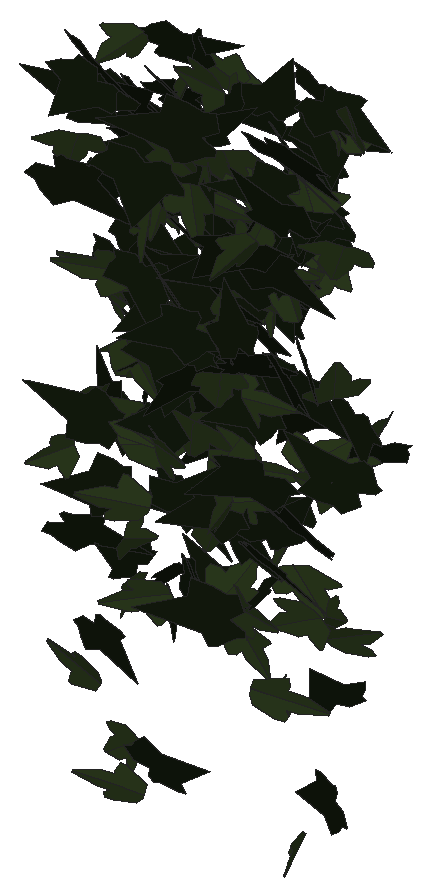
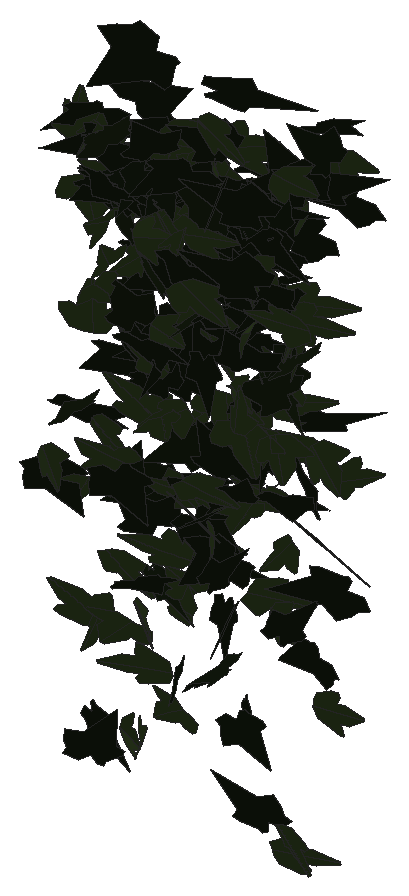
# SketchUp Ruby script. Lengths in millimetres.
U = 1.mm
M = Sketchup.active_model
def pt(a) = Geom::Point3d.new(a.map { |v| v * U })
def face(e, loops, mat)
  f = e.add_face(loops[0].map { |a| pt(a) })
  loops[1..].each { |l| e.add_face(l.map { |a| pt(a) }).erase! }
  f.material = f.back_material = mat if mat
  f
end
# faces: each face lists its corners as indices into pts; further lists are holes
def faces(e, pts, list, mat = nil) = list.each { |f| face(e, (f[0].is_a?(Array) ? f : [f]).map { |l| l.map { |i| pts[i] } }, mat) }
# xy, xz, yz: faces in a plane at the given z, y or x. An outline is a flat list of corners, or four numbers for a rectangle; further outlines are holes
def ring(l) = l.size == 4 ? [[l[0], l[1]], [l[2], l[1]], [l[2], l[3]], [l[0], l[3]]] : l.each_slice(2).to_a
def flat(e, list, mat, &to3) = list.each { |f| face(e, (f[0].is_a?(Array) ? f : [f]).map { |l| ring(l).map { |u, v| to3.(u, v) } }, mat) }
def xy(e, z, list, mat = nil) = flat(e, list, mat) { |x, y| [x, y, z] }
def xz(e, y, list, mat = nil) = flat(e, list, mat) { |x, z| [x, y, z] }
def yz(e, x, list, mat = nil) = flat(e, list, mat) { |y, z| [x, y, z] }
def lines(e, pts, list) = list.each { |a, b| e.add_line(pt(pts[a]), pt(pts[b])) }
# prism: a flat outline (further loops are holes) pulled along v
def prism(e, loops, v, mat = nil)
  f = face(e, loops, mat); d = Geom::Vector3d.new(v.map { |x| x * U })
  f.pushpull(f.normal.samedirection?(d) ? d.length : -d.length)
end
def box(e, o, s, mat = nil) = prism(e, [[o, [o[0] + s[0], o[1], o[2]], [o[0] + s[0], o[1] + s[1], o[2]], [o[0], o[1] + s[1], o[2]]]], [0, 0, s[2]], mat)
def at(x, y, z, deg = 0) = Geom::Transformation.translation(pt([x, y, z])) * Geom::Transformation.rotation(ORIGIN, Z_AXIS, deg.degrees)
def axes(o, x, y, z) = Geom::Transformation.new([*x, 0, *y, 0, *z, 0, *pt(o).to_a, 1])
def part(name) = M.definitions.add(name)
# library, detail: a bought-in or finely detailed component or shape, given as its bounding box
def library(name, o, s) = part(name).tap { |d| box(d.entities, o, s) }
def detail(e, o, s) = box(e.add_group.entities, o, s)
def put(e, d, t, mat = nil) = e.add_instance(d, t).tap { |i| i.material = mat if mat }
def group(e, t, mat = nil) = e.add_group.tap { |g| g.transformation = t; g.material = mat if mat }.entities
root = M.entities
M.materials.add("efeu1").color = [18, 25, 13]
M.materials.add("efeu2").color = [43, 57, 29]
c1 = part("ivyleaf_10")
p = [[0,12.8,-0.8],[-1.5,51.3,-10.9],[-4.9,51,-11.6],[-13.6,26.5,-7.3],[-13.2,15.9,-4.6],[-21.1,19.3,-7.2],
  [-29.5,16.3,-8.3],[-29.2,8.3,-6.2],[-19.7,-9.8,0.5],[-7.6,-13,4],[1,-12.2,5.8],[-0.4,51.1,-11.1],
  [-1.5,51.1,-10.9],[1,-12.4,5.9],[16.9,-12.4,3.5],[35.1,9.1,-5.1],[35,12.9,-6.1],[20.5,16.4,-4.9],
  [15.8,15,-3.8],[15.3,27.6,-7.1],[12.8,31.3,-7.8]]
faces(c1.entities,p,[[0,1,2,3,4,5,6,7,8,9,10],[11,12,0,13,14,15,16,17,18,19,20]],"efeu2")
c2 = part("ivyleaf_9")
p = [[39.1,54.8,31.7],[34.5,51.8,30.2],[-5.3,25.2,17.3],[-17.9,28.3,20.9],[-21.6,21.7,17],[-20.2,4.3,5.3],
  [-22.9,-0.3,2.5],[-17.1,-4,-0.6],[-2,-2.1,-1.2],[-0.7,-15.4,-10.1],[16.6,-22.3,-16.7],[21.1,-15.1,-12.5],
  [32.7,-10.7,-11],[46.1,-1.8,-6.6],[30.8,11.2,3.8]]
faces(c2.entities,p,[[0,1,2,3,4,5,6,7,8,9,10,11,12,13,14]],"efeu1")
put(root,c1,axes([3959.3,865.1,1629.4],[-0.5188,-0.54875,0.84407],[-0.22094,-0.8515,-0.59107],[1.90331,-0.24842,0.16146]))
put(root,c1,axes([3980.2,743.2,691],[-0.45175,0.21284,-0.91602],[-1.44478,0.51427,0.3162],[1.05644,0.79433,0.04073]))
put(root,c1,axes([3965.8,850.5,533.4],[1.04762,-0.60703,-0.60546],[-0.73059,0.46885,-0.81907],[1.45903,0.67064,0.02459]))
put(root,c1,axes([3920,890.6,1409.7],[-0.39414,-0.01153,-0.95363],[1.73672,-0.28603,-0.19471],[-0.52755,-0.933,0.07148]))
put(root,c2,axes([3991.9,777.8,1569.6],[-0.28849,0.0607,1.14922],[-2.18862,-0.05262,-0.1489],[0.08433,-1.15798,0.06701]))
put(root,c2,axes([3975.1,796.3,1081.1],[0.12478,0.00613,1.16954],[-0.12199,1.16963,-0.00254],[-2.22255,-0.06386,0.0658]))
put(root,c2,axes([3971.7,955.8,765.4],[-0.31084,0.75727,-0.51997],[0.19505,-0.5098,-0.77466],[-1.73736,-0.19272,0.00606]))
put(root,c1,axes([3972.5,705.2,1058.3],[0.21292,0.15716,-1.04889],[-0.94197,-0.92508,-0.1914],[-1.78526,0.50685,-0.0241]))
put(root,c1,axes([3990.2,821.5,481.6],[0.24968,0.09856,0.91362],[-1.44052,-0.51174,0.16389],[0.99172,-0.76814,0.00805]))
put(root,c1,axes([3973.4,764.7,1120.4],[-0.19767,-1.14603,0.30004],[-0.0368,-0.29951,-1.1507],[2.25434,-0.10538,0.00753]))
put(root,c1,axes([3970.4,827.9,1355.5],[0.48526,-0.30388,-1.02495],[0.00398,1.05383,-0.31193],[2.03461,0.07042,0.24507]))
put(root,c2,axes([3937.3,754.8,906.7],[0.32283,0.21121,-0.96973],[0.96693,0.82663,0.26891],[1.6226,-0.53463,0.03269]))
put(root,c2,axes([3944.2,782.7,1631.3],[0.53927,-0.56852,0.83965],[0.67816,-0.76039,-0.6351],[1.80678,0.45509,-0.01223]))
put(root,c2,axes([4014.9,757.6,987.8],[-1.56685,0.75225,0.36065],[-0.55985,0.21237,-1.11449],[-1.48572,-0.87335,0.03962]))
put(root,c1,axes([3986,845.9,1170.5],[-0.89079,-0.97271,-0.03245],[0.05811,0.02131,-1.07931],[1.85138,-0.46869,0.01827]))
put(root,c1,axes([3987.7,892.9,1483.1],[-0.11806,-0.85719,0.53445],[0.0114,-0.53576,-0.8586],[1.9225,-0.04946,0.03791]))
put(root,c2,axes([3966,828.1,1304.4],[0.14063,-1.03369,0.34224],[0.08121,-0.34001,-1.03619],[2.07076,0.08354,0.01739]))
put(root,c2,axes([3973.7,899,1446.5],[-1.18222,0.17725,0.73217],[1.18572,-0.41261,0.62845],[0.80599,0.867,0.1494]))
put(root,c2,axes([3950.4,953.6,1498.3],[0.57315,-0.22264,0.87712],[1.71725,0.00334,-0.30895],[0.13142,0.92737,0.21169]))
put(root,c1,axes([4024.5,759.8,1327.3],[-0.16228,0.03151,-1.04796],[-1.99092,-0.07288,0.08292],[-0.13345,1.0489,0.03725]))
put(root,c2,axes([3985.2,830,1076.9],[-1.15832,-0.62712,-0.2686],[0.35475,0.19339,-0.8739],[1.249,-0.63652,-0.00089]))
put(root,c1,axes([4002.9,904.7,1473.6],[0.31414,-0.4115,-0.84591],[-0.55598,0.79395,-0.44322],[1.7018,0.33534,0.01135]))
put(root,c2,axes([4022.5,859.4,1518.9],[0.01221,0.09272,-1.01055],[-1.83432,-0.31575,-0.03509],[-0.6045,0.95998,0.08606]))
put(root,c2,axes([4002.3,818.7,839.9],[0.25264,0.09874,0.93701],[-1.38172,-0.59242,0.16528],[1.14297,-0.738,-0.00731]))
put(root,c2,axes([4000.5,982.4,1000.1],[0.03816,-0.01733,0.94339],[-1.19837,-0.703,0.00047],[1.33741,-0.62942,-0.0265]))
put(root,c2,axes([4014.4,884.1,743.2],[0.20682,0.00701,-0.96456],[-1.64727,0.42917,-0.09439],[0.81034,0.87063,0.0543]))
put(root,c1,axes([3986.6,916.8,1097.2],[0.736,0.88073,0.19755],[0.1551,0.17997,-0.96189],[-1.71084,0.3952,-0.00222]))
put(root,c2,axes([4007.7,723.2,1639.6],[-1.20806,-0.67927,0.40065],[-0.471,-0.31675,-0.92912],[1.42509,-0.68051,0.03256]))
put(root,c2,axes([3972.5,844.6,1498.5],[1.54358,0.26888,0.39363],[0.69227,0.15304,-0.85399],[-0.5864,0.88843,0.02797]))
put(root,c1,axes([4007.5,682.2,1566.9],[-1.41854,-0.74022,0.08376],[-0.11277,-0.05921,-1.05046],[1.41328,-0.7477,0.00026]))
put(root,c1,axes([4035.5,740.3,1344],[-0.03682,-0.00566,-1.13432],[-1.94851,-0.48838,0.0199],[-0.92952,1.02399,0.00322]))
put(root,c2,axes([3981.5,970.6,857.2],[0.86654,-0.8092,-0.15571],[-0.14488,0.13584,-0.92849],[1.56161,0.46162,0.00026]))
put(root,c1,axes([4010.8,762.3,1289.9],[-0.55669,0.59897,0.81223],[-0.69346,0.72593,-0.66655],[-1.79114,-0.46721,0.00562]))
put(root,c2,axes([3966.7,923.5,1595.4],[0.35313,-0.02317,0.97755],[1.85352,-0.08478,-0.18686],[0.16675,0.99139,0.00686]))
put(root,c2,axes([3974.5,801.1,1575.2],[2.06075,-0.09705,-0.23007],[0.45128,0.07867,1.08275],[-0.14898,-1.10415,0.09737]))
put(root,c1,axes([4017.1,880.4,1358.7],[0.00474,0.6236,-0.76732],[-0.28991,0.7584,0.61586],[1.85935,0.11666,0.09798]))
put(root,c2,axes([3983.6,856.4,1541.6],[0.11582,-0.4186,0.95953],[0.59879,-0.9094,-0.41669],[1.90028,0.31207,0.07282]))
put(root,c2,axes([4040.2,703.4,1127.9],[-1.0054,-0.84373,-0.40503],[-0.35276,-0.36157,0.99495],[-1.74595,0.55892,0.03221]))
put(root,c1,axes([4035.1,981.4,1148.1],[0.96134,0.24095,-0.77105],[-1.36113,-0.28945,-0.55897],[-0.71488,0.87514,0.02741]))
put(root,c2,axes([4027.6,817.5,1143.6],[0.01757,0.05,-1.03786],[-1.46352,0.69835,0.02681],[1.32996,0.76782,0.04321]))
put(root,c1,axes([4046.4,971,1551.7],[0.7857,0.08387,0.85888],[-1.59559,-0.1867,0.4212],[0.3893,-0.93448,-0.00706]))
put(root,c2,axes([3993.1,745,771],[-0.34449,-0.05084,-0.95511],[1.80333,0.12305,-0.18612],[0.24829,-0.96429,0.02661]))
put(root,c2,axes([3982.2,676.6,1511.3],[0.1515,-0.21733,-1.11977],[1.78305,0.65277,-0.06009],[1.23837,-0.91329,0.22351]))
put(root,c2,axes([3992.3,752.7,1479.1],[0.52878,0.29984,-0.99452],[0.71031,0.93192,0.38524],[1.84491,-0.44474,0.13673]))
put(root,c2,axes([4009.4,916,1091.5],[-0.27308,-0.21788,0.95466],[1.55252,0.50714,0.23835],[-1.03092,0.82145,0.10606]))
put(root,c2,axes([4013.2,799.1,1391.5],[0.42792,-0.41087,-1.00066],[-0.5291,0.96576,-0.45901],[1.98959,0.3452,0.09315]))
put(root,c2,axes([3992.6,881.6,1568.5],[1.50869,-0.67716,0.24411],[0.35844,-0.15536,-1.04255],[1.32222,0.81477,0.00409]))
put(root,c2,axes([4009.9,925,1009.6],[1.40511,0.54308,0.36462],[0.55207,0.22099,-0.9165],[-1.11583,0.79321,0.0057]))
put(root,c1,axes([4047.3,850.1,1171.6],[-2.10997,0.00574,0.38048],[-0.72416,-0.00251,-1.10865],[-0.00879,-1.17211,0.00423]))
put(root,c2,axes([3994.4,819.9,1241.7],[1.21504,-0.80467,0.3748],[0.50445,-0.2678,-1.02644],[1.61235,0.69017,0.03869]))
put(root,c2,axes([4020.4,981.5,1097.9],[-0.30074,-0.9049,0.23974],[-0.09171,-0.23495,-0.91856],[1.77925,-0.16506,-0.00683]))
put(root,c2,axes([4033.6,913.4,1613],[0.58197,-0.11355,-0.91049],[-1.26157,0.63625,-0.30197],[1.20744,0.7195,0.12334]))
put(root,c2,axes([4003.5,778,1264.8],[1.67676,-0.58861,-0.09034],[-0.12402,0.06506,-1.05941],[1.12656,0.88325,0.01784]))
put(root,c1,axes([4030.3,889,1567.8],[0.72251,-0.89473,0.17404],[0.15816,-0.15377,-0.9718],[1.72754,0.38828,0.01618]))
put(root,c2,axes([4059,801.5,1514.5],[-0.98542,-0.25859,0.76669],[-1.34808,-0.29511,-0.57789],[0.74435,-0.87682,-0.03161]))
put(root,c1,axes([4047.5,923.3,1025.3],[0.10702,-0.09961,0.98424],[-1.07951,0.80445,0.11382],[-1.54257,-0.56987,-0.01137]))
put(root,c1,axes([4003.9,744.4,1111.6],[0.93535,0.48869,0.89138],[1.18993,0.63537,-0.69305],[-1.52549,0.79524,0.00595]))
put(root,c1,axes([4035.6,785.5,839.4],[0.27271,-0.90028,0.5439],[0.25623,-0.52871,-0.91061],[1.98536,0.1919,0.04281]))
put(root,c2,axes([4058.5,758.6,1214.1],[-0.4518,0.92759,0.36764],[-0.17051,0.35656,-0.95748],[-1.89132,-0.25373,-0.0015]))
put(root,c1,axes([4024.3,747.9,1512.6],[-0.90522,0.829,-0.60657],[0.59387,-0.52025,-0.9557],[-1.86262,-0.56876,-0.00992]))
put(root,c1,axes([4035.4,875.9,1203],[-1.30905,0.62472,0.39731],[0.55759,-0.26837,0.92917],[1.29403,0.74761,0.00155]))
put(root,c2,axes([4034.2,855.2,1291.9],[-1.1481,-0.14236,0.71503],[1.3556,0.08292,0.61743],[-0.29603,0.93182,0.05429]))
put(root,c1,axes([4044,824.8,1156.3],[-1.55833,-0.68303,-0.25266],[0.37039,0.16114,-1.06628],[1.33562,-0.8416,0.0009]))
put(root,c2,axes([4072.6,921.7,777.9],[-0.79872,-0.82739,0.35569],[0.29237,0.3209,0.92771],[-1.68891,0.44684,-0.00762]))
put(root,c1,axes([4050.5,742.7,931.9],[-0.26613,-0.38674,-0.93422],[0.59974,0.87947,-0.41125],[1.82849,-0.34475,-0.00108]))
put(root,c2,axes([4025.7,825.2,526.5],[-0.01457,0.02402,0.95368],[1.32773,-0.65036,0.02198],[1.23839,0.69756,-0.01235]))
put(root,c1,axes([4052.1,808.4,1424.9],[1.18227,-0.77185,0.22562],[0.28592,-0.16868,-0.99072],[1.50351,0.63901,0.01099]))
put(root,c1,axes([4020.8,797.8,1043.3],[1.01431,-0.22774,-0.89789],[1.75743,0.0486,0.53577],[-0.13957,-1.04301,0.22102]))
put(root,c2,axes([4076,904.1,1301],[0.8911,-0.05599,-0.8817],[-1.63125,0.2132,-0.46869],[0.40776,0.97528,0.05184]))
put(root,c1,axes([4091.1,755,848.1],[0.54036,0.20306,-1.03576],[-1.59962,-0.60529,-0.34906],[-1.21508,0.88715,-0.00108]))
put(root,c1,axes([4065.8,969.7,1550.4],[0.23464,0.93867,-0.15253],[-0.06358,-0.14943,-0.94664],[-1.80879,0.12702,0.01349]))
put(root,c2,axes([4077.8,889.4,1554],[0.50407,0.77888,0.57502],[0.35612,0.54372,-0.82268],[-1.80783,0.32428,-0.00173]))
put(root,c2,axes([4053.5,807.6,1438.7],[-0.92735,0.16597,1.02057],[1.73071,-0.46816,0.5103],[0.93655,1.02947,0.06753]))
put(root,c2,axes([4092.2,900.2,1036.4],[-0.10703,0.43277,-0.84754],[0.06019,-0.84769,-0.43495],[-1.81015,-0.05378,0.03565]))
put(root,c1,axes([4045.7,750.8,1218],[1.30161,-0.27451,0.95007],[1.70821,-0.3127,-0.73644],[0.79024,1.12809,0.02706]))
put(root,c1,axes([4078.7,820.4,1088],[-0.58132,-0.87118,-0.03194],[-0.0202,-0.03012,0.92317],[-1.65901,0.30563,-0.00005]))
put(root,c2,axes([4087.5,911.1,1041.8],[-1.30778,0.71498,-0.02906],[-0.0586,0.01071,0.99154],[1.36062,0.68768,0.01477]))
put(root,c1,axes([4084.9,815.6,1212.4],[0.40159,-0.79797,0.49323],[0.29082,-0.46957,-0.82506],[1.76155,0.25944,0.02377]))
put(root,c2,axes([4087.3,823.6,849],[0.71431,-0.38393,-0.85916],[-1.14458,0.61358,-0.53691],[1.37753,0.7089,-0.0006]))
put(root,c1,axes([4113.7,893,1402.1],[-1.15489,-0.47004,0.63147],[-0.96006,-0.37991,-0.76754],[1.15017,-0.78908,-0.00661]))
put(root,c2,axes([4070.4,849.1,1097.7],[-0.89777,-0.03829,0.85441],[1.38276,-0.53275,0.37725],[0.85881,0.81775,0.28577]))
put(root,c2,axes([4103.5,821.8,852.7],[0.84581,-0.11014,-0.90603],[-1.6166,0.31882,-0.4554],[0.63559,0.95747,0.04741]))
put(root,c2,axes([4082.5,742,1362.8],[-0.50687,-1.07412,-0.0713],[0.04352,0.06779,-1.10662],[2.04829,-0.26724,0.00587]))
put(root,c2,axes([4098.8,765.6,1300],[0.21039,-0.41617,-1.00154],[0.46241,-0.97164,0.43056],[-2.01169,-0.26687,-0.00578]))
put(root,c2,axes([4073.2,773.6,1339.5],[-0.47434,0.02793,0.93591],[1.72672,-0.23219,0.24853],[0.44048,0.94028,0.03357]))
put(root,c1,axes([4085.3,736.5,1448.4],[1.02341,-0.67256,0.75229],[0.85409,-0.60411,-0.86086],[1.72014,0.7001,-0.02014]))
put(root,c2,axes([4096.9,718.3,1541.2],[-1.18243,-0.96049,-0.15125],[0.15929,0.126,-1.14391],[1.84366,-0.62689,0.00183]))
put(root,c1,axes([4097.5,977,1231.1],[0.66283,0.84637,-0.28373],[-0.20548,-0.26238,-0.91523],[-1.68644,0.36462,0]))
put(root,c1,axes([4133.7,819.6,1632.9],[0.50574,-0.19376,-1.04021],[-1.36764,0.75419,-0.32406],[1.47813,0.7641,0.05607]))
put(root,c2,axes([4108.7,788.4,999.5],[0.41984,-0.71775,-0.75354],[0.48759,-0.70912,0.75044],[-1.91964,-0.3371,0.02581]))
put(root,c2,axes([4129.4,876,1077.8],[-1.56644,-0.47534,0.30066],[-0.49927,-0.14695,-0.95045],[0.94689,-0.86384,-0.00376]))
put(root,c1,axes([4147.8,732.4,1559.2],[-1.19547,0.36275,-0.8921],[-1.46589,0.45013,0.72535],[1.10023,0.99387,-0.00291]))
put(root,c2,axes([4132.1,753.7,1135.3],[-0.57594,-0.34038,1.09723],[-1.40365,-0.81241,-0.45543],[1.67637,-0.79718,-0.00437]))
put(root,c2,axes([4101.6,934.9,777.7],[0.25375,-0.15782,-0.98314],[1.48344,-0.60072,0.20214],[-1.17928,-0.78961,0.04273]))
put(root,c1,axes([4135,829.2,948.9],[-1.2988,-0.84989,0.07287],[-0.08314,-0.05837,-1.08996],[1.62131,-0.68382,0.00248]))
put(root,c2,axes([4131.4,914.2,1333.9],[0.48913,-0.90153,-0.3941],[0.22067,-0.37674,0.93742],[-1.85953,-0.28185,0.00758]))
put(root,c1,axes([4132.7,937.3,1351.2],[-0.0358,-0.66501,0.68277],[0.01748,-0.683,-0.66498],[1.81387,-0.00654,0.01989]))
put(root,c2,axes([4124.3,710.3,1392.4],[1.40679,-0.3417,-0.62969],[-1.073,0.28083,-0.8142],[0.84133,0.92953,0.01451]))
put(root,c1,axes([4134.6,804.9,1270.4],[1.5576,-0.56988,-0.2026],[-0.29497,0.1319,-0.99709],[1.11266,0.83273,0.01929]))
put(root,c1,axes([4159.4,618.3,1076.9],[0.14102,0.27954,1.0388],[-0.94969,-0.91353,0.28142],[1.81379,-0.50005,0.06658]))
put(root,c1,axes([4109.6,919.9,719.5],[1.3014,-0.17805,0.68953],[1.2916,-0.1268,-0.70575],[0.41078,0.96278,0.03457]))
put(root,c1,axes([4142.6,856.8,1058.7],[1.8977,-0.36879,-0.24772],[-0.42754,0.10659,-1.06291],[0.72948,1.02188,0.02147]))
put(root,c2,axes([4110.3,800.8,1399.4],[1.60916,-0.26924,-0.63782],[1.12677,-0.24068,0.88642],[-0.683,-1.03139,-0.04035]))
put(root,c2,axes([4145.3,959.8,1336.7],[-1.58385,-0.32565,-0.35437],[0.63283,0.12271,-0.89363],[0.6622,-0.89615,0.00641]))
put(root,c1,axes([4111.6,925.4,980.3],[-0.37019,-0.09506,0.98352],[1.56689,0.5387,0.21489],[-1.03988,0.84555,-0.02633]))
put(root,c2,axes([4142.5,903.6,1292.6],[0.40633,-0.33568,-0.92615],[-0.93997,0.78348,-0.39782],[1.62221,0.53806,0.00147]))
put(root,c2,axes([4130.2,762.3,1520.7],[-0.4223,-0.87568,-0.56529],[0.3186,0.54052,-0.903],[1.95793,-0.27682,0.02501]))
put(root,c2,axes([4145.9,744.4,1251.9],[-1.57213,-0.82852,-0.24431],[0.33429,0.16986,-1.16995],[1.60961,-0.8445,0.00436]))
put(root,c1,axes([4119,722.1,1104.4],[-0.81597,0.09254,1.03856],[1.7009,-0.54581,0.41757],[1.02217,0.98209,0.13421]))
put(root,c1,axes([4159.8,752,1139.4],[-2.05521,-0.00447,0.20463],[-0.38938,-0.00803,-1.07986],[0.0112,-1.09906,0.00705]))
put(root,c2,axes([4162.4,803,1243.9],[0.33297,-0.63504,0.84748],[-0.25241,0.83907,0.65611],[-1.99964,-0.21166,0.0583]))
put(root,c2,axes([4125.5,877.3,1589.2],[-0.11988,-0.31077,-1.01968],[0.52624,0.98174,-0.31629],[1.95935,-0.28269,0.02256]))
put(root,c2,axes([4132.3,843.9,1332.8],[0.14937,-1.1817,-0.18202],[-0.02935,0.1814,-1.1843],[2.27535,0.07991,-0.00333]))
put(root,c2,axes([4157.7,959.1,935.4],[-1.05387,-0.77052,0.15859],[-0.17214,-0.13029,-0.94885],[1.48726,-0.56107,0.00255]))
put(root,c2,axes([4197.5,711.7,1625.2],[-1.33243,-0.05021,0.93375],[-1.76909,-0.08969,-0.70176],[0.19385,-1.16361,0.0138]))
put(root,c1,axes([4164.6,942.2,874.8],[0.69109,-0.90909,-0.12377],[-0.09415,0.11352,-0.97893],[1.74361,0.36646,-0.0038]))
put(root,c1,axes([4145.2,784.1,1497.5],[-1.37136,-0.22656,-0.62415],[1.12253,0.20465,-0.7552],[0.58043,-0.93106,-0.01412]))
put(root,c2,axes([4144.4,778.1,1579.3],[-0.05581,-0.01886,0.99555],[1.66718,0.47306,0.03476],[-0.90102,0.87647,0.00266]))
put(root,c2,axes([4154.2,842.2,1406],[-1.37944,-0.13793,-0.87148],[1.61477,0.20057,-0.73739],[0.46086,-1.11561,-0.02483]))
put(root,c2,axes([4161.1,728.1,1023.3],[-1.11741,-0.05013,0.79979],[1.51699,0.06588,0.58926],[-0.15753,0.98997,0.00129]))
put(root,c1,axes([4134.1,781,1483.3],[-0.0525,-0.06474,-1.11764],[2.0184,-0.35961,-0.00535],[-0.68247,-1.05857,0.07016]))
put(root,c1,axes([4160.9,857.5,1168.8],[-0.41114,-0.26819,-0.96426],[1.05518,0.78922,-0.34372],[1.58588,-0.59464,-0.02129]))
put(root,c2,axes([4149.4,846.1,1208.8],[-0.00512,-0.16357,0.98202],[0.88986,-0.86719,-0.14316],[1.67277,0.46082,0.07916]))
put(root,c1,axes([4154.4,780.4,1547.6],[0.18232,-0.09945,1.12868],[1.3919,-0.85972,-0.13782],[1.64706,0.73755,-0.00847]))
put(root,c1,axes([4165.4,818.2,857.9],[0.97125,0.60104,-0.65119],[0.8034,0.49583,0.78846],[1.4829,-0.66229,-0.00066]))
put(root,c2,axes([4222.7,741.9,865.4],[-1.62417,0.08103,0.70567],[-1.33677,0.06808,-0.85723],[-0.20141,-1.10527,-0.00107]))
put(root,c1,axes([4173.5,931.5,654.2],[-0.01833,0.24464,-0.92655],[0.10711,-0.92485,-0.24478],[-1.8207,-0.05687,-0.00507]))
put(root,c1,axes([4207.5,881.9,1454.2],[-0.64367,0.54046,-0.77229],[-1.0865,0.53546,0.62473],[1.42755,0.65122,0.12726]))
put(root,c2,axes([4195.5,705.3,1255],[-0.32404,0.68314,-0.9242],[0.33745,-0.90749,-0.70345],[-2.1611,-0.24413,0.02873]))
put(root,c2,axes([4157.2,889.4,1230.9],[0.27826,-0.34802,0.88683],[0.62463,-0.82389,-0.37743],[1.70213,0.35924,-0.00647]))
put(root,c2,axes([4170,835.6,946.5],[0.99524,-0.72251,-0.61524],[-0.60159,0.52973,-0.89076],[1.70293,0.60939,0.04488]))
put(root,c2,axes([4197.4,886.1,1410.5],[-1.32954,0.48635,-0.46952],[0.71273,-0.2837,-0.85104],[-1.07112,-0.79245,0.01651]))
put(root,c1,axes([4164.8,731,1511.6],[1.6932,-0.48685,0.6537],[1.08888,-0.31622,-1.01416],[1.10487,1.05775,-0.00231]))
put(root,c1,axes([4158,912.5,1275.5],[0.60157,-0.22187,-0.94561],[1.43474,-0.57099,0.38596],[-1.16561,-0.81734,-0.01294]))
put(root,c2,axes([4206.1,943.5,1088.8],[0.22107,0.74175,-0.59653],[-0.16495,-0.59022,-0.75077],[-1.80406,0.14486,-0.00445]))
put(root,c2,axes([4195.2,873.3,1598],[-0.82609,-0.33463,0.84206],[1.36391,0.44459,0.54608],[-1.05532,0.83654,0.04661]))
put(root,c2,axes([4204.3,744.9,1333.4],[-1.86316,-0.10643,0.69661],[1.31595,0.08506,0.9847],[-0.25886,1.1985,-0.00803]))
put(root,c2,axes([4221,833.6,869.8],[-0.98447,0.78347,-0.3447],[0.37744,-0.28209,-0.93878],[-1.58471,-0.5539,-0.00946]))
put(root,c1,axes([4207.8,759.1,1575.5],[-1.69086,-0.62522,-0.23962],[0.37213,0.13851,-1.08637],[1.21876,-0.90969,-0.00073]))
put(root,c1,axes([4173.6,827.3,825.8],[-0.45687,0.07296,1.05185],[1.91807,-0.30115,0.2509],[0.58973,1.03601,-0.00115]))
put(root,c2,axes([4174.4,763.7,1349.1],[0.55885,-0.36188,0.86209],[1.01084,-0.67909,-0.46597],[1.46443,0.60685,-0.00735]))
put(root,c1,axes([4178.7,808,1004.3],[0.53255,0.08284,-0.88496],[1.57603,0.31279,0.29112],[0.6146,-0.87386,0.02031]))
put(root,c2,axes([4191.5,778.9,1069.6],[1.67644,-0.42555,-0.01649],[-0.02114,0.01493,-0.97822],[0.81024,0.88088,0.00861]))
put(root,c2,axes([4199.1,894.7,1268.6],[-0.26301,0.21278,0.98147],[0.49471,-0.94938,0.24243],[1.8462,0.28471,0.07486]))
put(root,c1,axes([4225.1,724.2,1248.9],[-1.3056,-0.72851,-0.02067],[0.04,0.0086,-1.00062],[1.38648,-0.68626,0.00941]))
put(root,c2,axes([4190.9,803.4,1370.5],[1.88514,0.13202,0.2585],[0.48758,0.03452,-0.99927],[-0.2597,1.02311,0.00036]))
put(root,c2,axes([4235.5,720.8,1049.8],[-0.05563,-0.38443,-0.92473],[-0.10658,-0.92304,0.3855],[-1.90298,0.06294,0.00544]))
put(root,c1,axes([4195.9,933.3,837.7],[1.59402,0.30136,0.48768],[0.87272,0.16602,-0.89011],[-0.65482,0.95486,0.00085]))
put(root,c2,axes([4214.7,872.7,1554.9],[1.38483,-0.3147,-0.63293],[-1.05863,0.30558,-0.7914],[0.8301,0.9147,0.04663]))
put(root,c2,axes([4227.7,976,632.9],[0.8205,0.27712,0.8202],[-1.40467,-0.36131,0.51001],[0.86128,-0.85326,0.05042]))
put(root,c1,axes([4209,816,1406.6],[1.85511,-0.54995,-0.13311],[0.23046,-0.05626,1.11913],[-1.05195,-0.98217,0.01043]))
put(root,c2,axes([4191.4,790.1,1233.1],[1.47486,0.33465,0.69773],[1.20983,0.2878,-0.84406],[-0.83985,1.00226,0.0094]))
put(root,c2,axes([4237.6,800.8,1174.3],[0.07899,-0.51476,-0.88394],[0.07641,-0.88316,0.5162],[-1.94529,-0.05559,-0.01562]))
put(root,c2,axes([4200.9,910,1334.2],[-0.10661,-0.42556,0.89771],[0.80492,-0.8238,-0.36413],[1.71088,0.36106,0.22725]))
put(root,c2,axes([4246.5,638.8,1372.3],[-0.25671,-0.4355,-0.98711],[-0.05877,-0.99283,0.44225],[-2.05255,0.08289,0.11079]))
put(root,c2,axes([4242.7,853.1,1195.9],[-0.07365,-0.71389,-0.7484],[0.06834,-0.7494,0.71298],[-1.96726,0.0007,0.05279]))
put(root,c1,axes([4205.3,868.7,1158.8],[-1.36966,-0.19837,0.80282],[1.4849,0.18989,0.74632],[-0.52169,1.06131,0.01653]))
put(root,c2,axes([4244.8,788.4,1489.7],[-0.44707,0.4171,-0.98366],[-1.18915,0.76336,0.47289],[1.64949,0.66336,0.07431]))
put(root,c2,axes([4223.1,833.2,954],[-0.5552,-0.26332,1.0162],[1.76397,0.43063,0.37765],[-0.93811,0.96557,0.1087]))
put(root,c1,axes([4238,720.1,1372.8],[0.97459,-1.05709,0.37701],[0.32884,-0.33521,-1.17456],[2.11052,0.54037,0.00891]))
put(root,c1,axes([4202.4,789.3,1187.4],[0.38212,-0.18276,-1.06134],[1.96984,-0.26562,0.24154],[-0.56644,-1.04699,0.12399]))
put(root,c2,axes([4283.3,727.6,1440.7],[-0.046,-0.06681,-1.27613],[-1.36833,-1.05448,0.06883],[-2.01062,0.71915,-0.01764]))
put(root,c1,axes([4237.7,782.6,1544],[1.51102,0.74825,0.04289],[0.05606,0.03128,-1.09096],[-1.4253,0.79448,0.00256]))
put(root,c1,axes([4244.9,710.5,1061.8],[0.00897,-0.14446,1.06579],[0.72674,-0.99615,-0.13671],[1.91361,0.37899,0.04692]))
put(root,c2,axes([4239.5,800,1375.3],[-0.98363,-0.34664,-0.82599],[1.31368,0.45369,-0.62229],[1.08662,-0.86228,0.00463]))
put(root,c1,axes([4224.6,828.8,708.2],[0.1746,0.07386,1.0205],[1.53159,0.62754,-0.11776],[-1.20257,0.80995,-0.00182]))
put(root,c2,axes([4236.2,929.5,1620.3],[0.23901,-0.97764,0.57358],[0.34407,-0.55242,-0.98117],[2.12962,0.19898,0.09415]))
put(root,c2,axes([4286.9,701.1,1487.7],[0.5959,0.62899,-0.95138],[-0.81944,-0.84839,-0.7026],[-2.00999,0.53235,0.00438]))
put(root,c1,axes([4266.5,910.5,810.2],[-0.06699,-0.59204,-0.8241],[0.33859,0.80822,-0.58823],[1.9013,-0.16479,0.07572]))
put(root,c1,axes([4258.5,815.5,1376.5],[-0.29461,-0.29786,-1.06539],[0.8536,0.96648,-0.33537],[1.92459,-0.47425,-0.01434]))
put(root,c1,axes([4275.1,903.9,1360.3],[0.56851,0.71869,-0.68187],[-0.55945,-0.61582,-0.77785],[-1.80057,0.41826,0.02639]))
put(root,c2,axes([4303.7,765.8,1547.3],[-0.98047,-0.15717,0.83954],[-1.49761,-0.29395,-0.53789],[0.63218,-0.94012,0.02783]))
put(root,c2,axes([4254.6,893.3,1528],[-0.89877,-0.264,-0.81745],[1.58004,0.09933,-0.51169],[0.41992,-0.93881,0.17573]))
put(root,c1,axes([4274.3,875.2,1386.9],[0.3218,0.77143,-0.57978],[0.28808,0.56013,0.78942],[1.81388,-0.22582,-0.02252]))
put(root,c1,axes([4265.6,783.8,1369.1],[1.14251,-0.63921,0.55004],[0.79561,-0.3608,-0.87554],[1.39387,0.72989,0.0489]))
put(root,c2,axes([4248,845.8,1533.3],[1.37051,-0.65789,0.31455],[0.43438,-0.21651,-0.97537],[1.31811,0.75539,-0.00562]))
put(root,c1,axes([4272.1,935.5,1050.7],[0.95865,0.80992,0.16445],[0.16496,0.13975,-0.95377],[-1.56422,0.51111,0.0002]))
put(root,c1,axes([4258.8,876.3,1063.6],[1.26497,0.29329,-0.82447],[1.23617,0.52846,0.71161],[1.11608,-0.91774,0.14628]))
put(root,c1,axes([4304.9,819.9,858.5],[1.35335,-0.24592,-0.67848],[-1.16172,0.30317,-0.74963],[0.73271,0.93491,0.06462]))
put(root,c1,axes([4275.5,742.8,1407.9],[-1.65136,-0.60628,-0.60262],[0.95485,0.33403,-1.05844],[1.31722,-1.00221,0.01177]))
put(root,c2,axes([4259.9,876,1589.7],[0.48083,0.07911,-1.00927],[0.52103,0.99612,0.14661],[1.85494,-0.3003,0.22044]))
put(root,c2,axes([4256.3,764.5,969.4],[1.87717,-0.53087,0.11326],[0.18974,-0.05374,-1.12011],[1.01552,0.99135,-0.00007]))
put(root,c1,axes([4295.8,833.9,1505.4],[1.74922,0.4527,0.16181],[-0.27985,-0.06766,1.02453],[0.87111,-0.93077,0.00422]))
put(root,c2,axes([4290.9,825.5,982.2],[1.41541,-0.64796,0.21808],[-0.29529,0.15387,0.98628],[-1.26722,-0.75959,0.01376]))
put(root,c2,axes([4265.2,831.4,1208.6],[-0.33453,-0.30886,-0.93652],[1.41266,0.58486,-0.33219],[1.23564,-0.75226,0.12624]))
put(root,c1,axes([4300.7,684,1500.3],[-0.15082,-0.77106,0.88087],[-0.02025,-0.88238,-0.77333],[2.22793,-0.06022,0.0526]))
put(root,c2,axes([4280.4,823.6,1423.5],[0.07079,0.90417,0.64244],[-0.13223,-0.63964,0.90425],[2.10682,-0.07053,0.03517]))
put(root,c2,axes([4300.3,842.6,1486.7],[-1.64645,-0.48561,-0.40044],[0.63355,0.22467,-0.9916],[1.01666,-0.92643,-0.03057]))
put(root,c2,axes([4292.8,876.9,1595.6],[-0.43131,-0.98888,-0.02007],[0.0098,0.01941,-1.01451],[1.88239,-0.22668,0.00068]))
put(root,c1,axes([4307.8,977.7,1098.5],[-0.03457,-0.98187,0.02449],[-0.00107,-0.02448,-0.98204],[1.86928,-0.01817,-0.00011]))
put(root,c2,axes([4316.8,959.1,1069.9],[0.2031,0.71295,-0.66483],[-0.116,-0.66262,-0.72036],[-1.85168,0.11971,-0.02779]))
put(root,c1,axes([4306,879.1,1587.9],[0.5127,-0.05167,-1.01039],[0.10401,1.04481,-0.03886],[1.92268,-0.04274,0.27153]))
put(root,c1,axes([4329.4,824.2,1071.3],[0.5648,-0.31387,-0.91382],[-1.16977,0.67628,-0.43189],[1.41889,0.68249,0.0077]))
put(root,c2,axes([4309.1,759.1,1269.8],[1.36301,-0.23395,-0.85494],[-1.54972,0.26057,-0.75341],[0.66645,1.0844,-0.00341]))
put(root,c1,axes([4309.9,879.6,1584.1],[1.63634,0.56003,0.1115],[-0.20974,-0.03502,1.02564],[1.06635,-0.86628,0.03062]))
put(root,c2,axes([4318.3,647.5,1370],[-0.83624,-0.68038,0.79048],[0.77214,0.67871,0.80969],[-1.82864,0.59772,-0.0196]))
put(root,c2,axes([4281.3,838.2,1491.2],[-0.40105,-0.35699,-0.92094],[1.29934,0.62785,-0.3996],[1.35845,-0.70593,0.11033]))
put(root,c1,axes([4309,839.7,1424.1],[0.42219,0.3763,-1.02635],[0.41567,1.0109,0.41784],[2.03856,-0.28406,0.12736]))
put(root,c2,axes([4289.1,878.3,1635.4],[0.28332,-0.50956,-0.86644],[0.36597,0.87415,-0.48106],[1.87771,-0.09349,0.22449]))
put(root,c2,axes([4346.3,821.6,586.6],[-0.00353,0.06279,-1.0646],[-2.01004,0.1476,0.01055],[0.2816,1.05432,0.06193]))
put(root,c1,axes([4330.2,749.2,1386],[-0.28906,1.1664,-0.31602],[-0.17423,0.30649,1.17521],[2.29332,0.1703,0.04945]))
put(root,c2,axes([4352.4,656,1172],[0.13551,0.10786,-1.10788],[-0.93719,-0.99255,-0.12828],[-1.89991,0.4973,-0.01574]))
put(root,c1,axes([4302.8,882.8,797.7],[-1.12193,-0.48417,0.65374],[1.17554,0.25903,0.7488],[-1.00761,0.8413,0.14568]))
put(root,c2,axes([4314.3,909.3,1140],[-0.01168,-0.93398,0.44385],[0.05778,-0.44383,-0.93352],[1.96721,0.00749,0.03005]))
put(root,c1,axes([4333.1,878.5,1600.4],[-1.61049,0.58583,0.16938],[0.25742,-0.10219,1.02918],[1.1317,0.85692,0.00694]))
put(root,c1,axes([4327.1,769.6,540.8],[0.55528,-0.70339,0.62013],[0.43197,-0.57717,-0.76145],[1.73161,0.36954,-0.00891]))
put(root,c2,axes([4294.3,719.6,1462.6],[-0.0125,-0.0431,-1.13577],[1.82891,0.6063,-0.02857],[1.15513,-0.96042,0.03294]))
put(root,c2,axes([4361.2,700.7,1546.9],[0.4808,-0.24003,1.001],[-1.45042,0.64925,0.34802],[-1.31695,-0.80268,-0.01784]))
put(root,c2,axes([4309.2,800.8,1281.6],[0.40328,-0.14882,-1.00993],[1.66767,-0.50267,0.25792],[-0.99678,-0.90121,0.02292]))
put(root,c2,axes([4378.8,825.7,1084.2],[-1.82034,-0.41932,-0.33083],[-0.5786,-0.1305,1.04434],[-0.83579,1.00361,-0.00243]))
put(root,c2,axes([4322.2,716.3,1650],[2.43682,-0.07869,-0.0774],[-0.14704,0.0047,-1.2828],[0.15003,1.28271,-0.00004]))
put(root,c1,axes([4366.1,817.3,1456.9],[-1.61002,-0.55385,0.1592],[-0.2424,-0.09609,-1.01108],[1.06965,-0.85542,0.0105]))
put(root,c1,axes([4357.5,815.3,1234.1],[-0.98899,-1.00295,-0.2604],[-0.23269,-0.22993,1.12957],[-1.95832,0.53383,-0.00271]))
